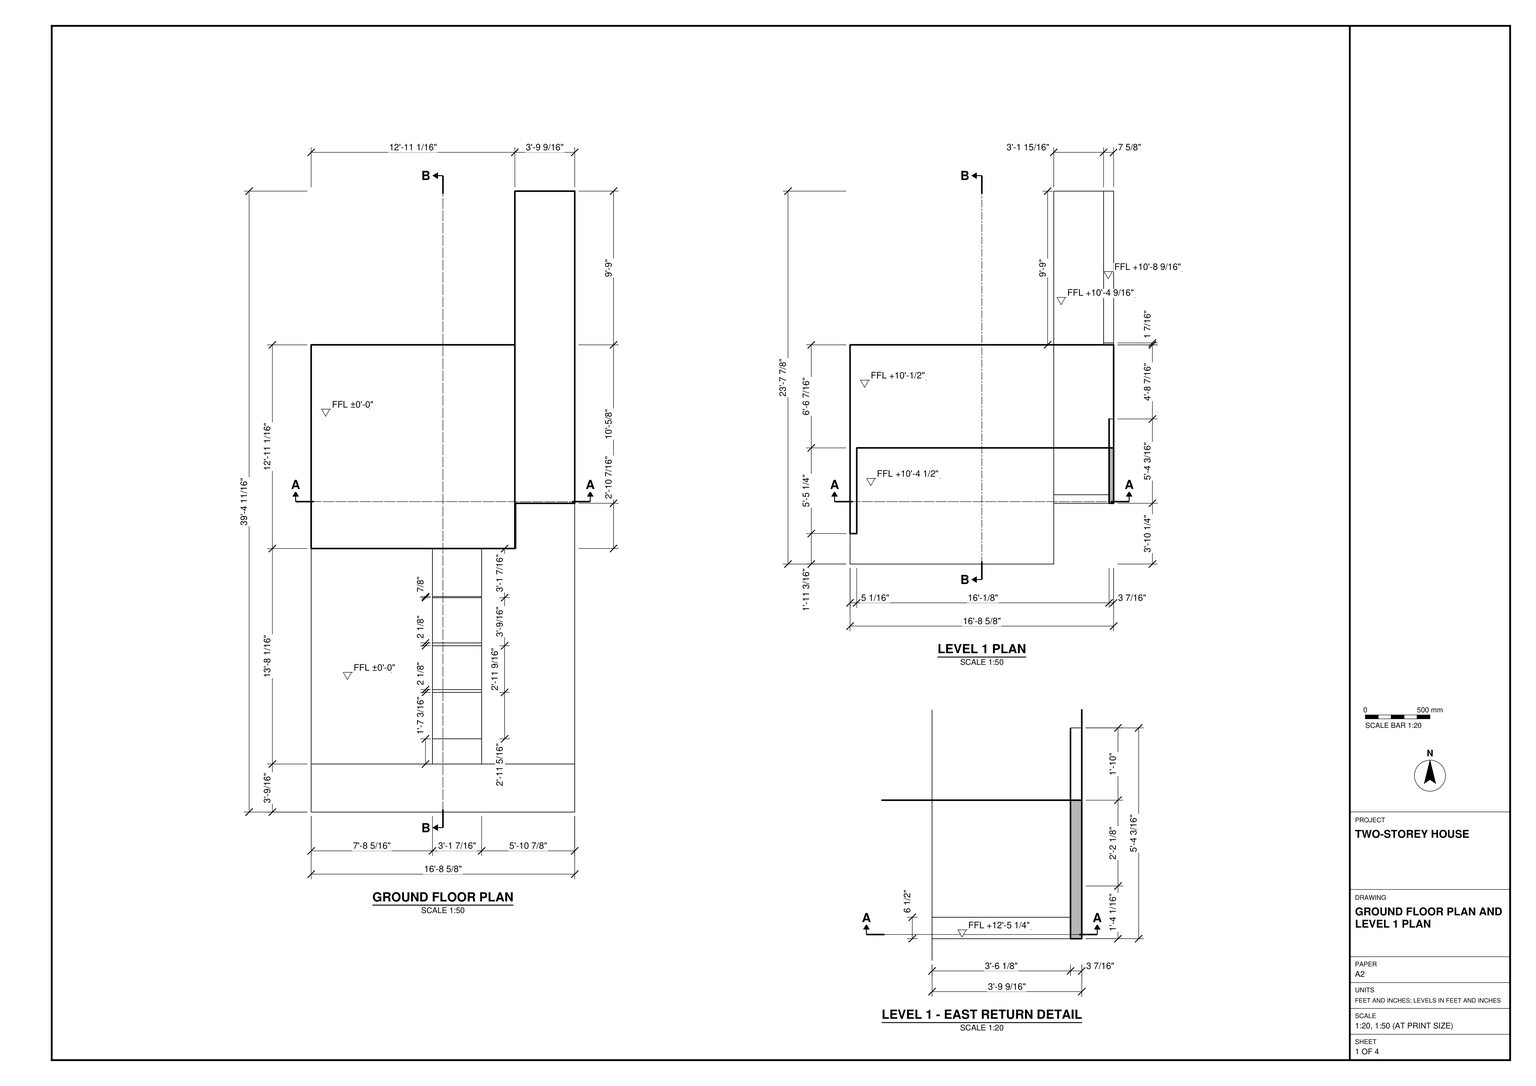
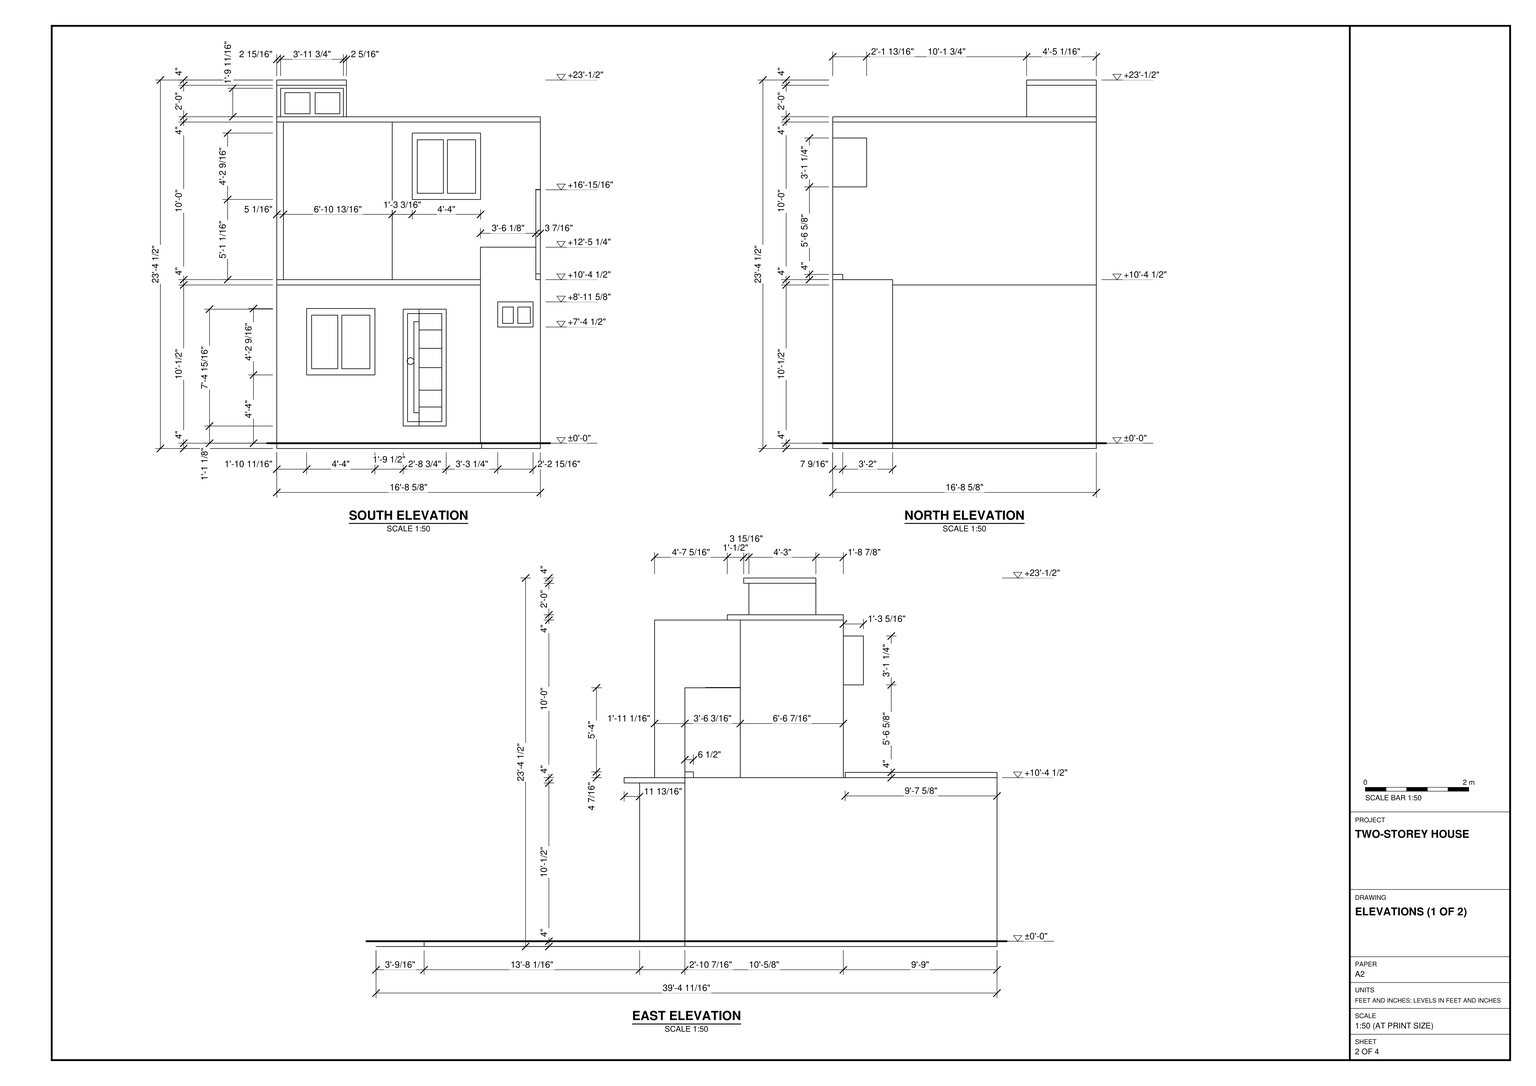
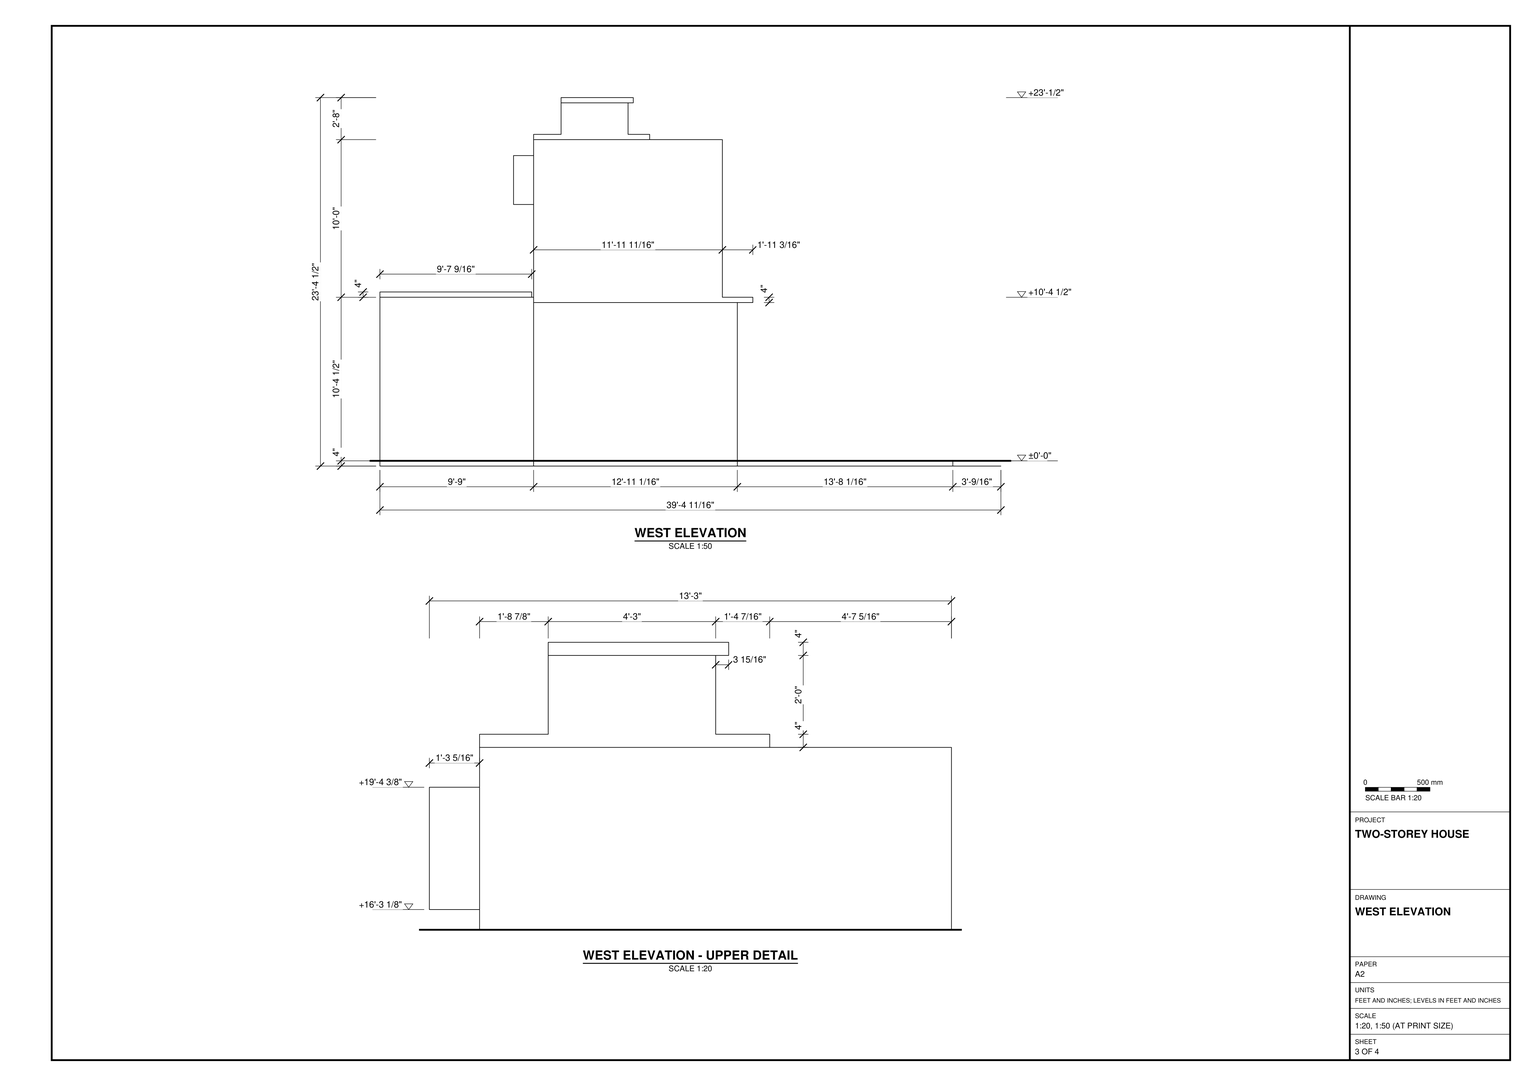
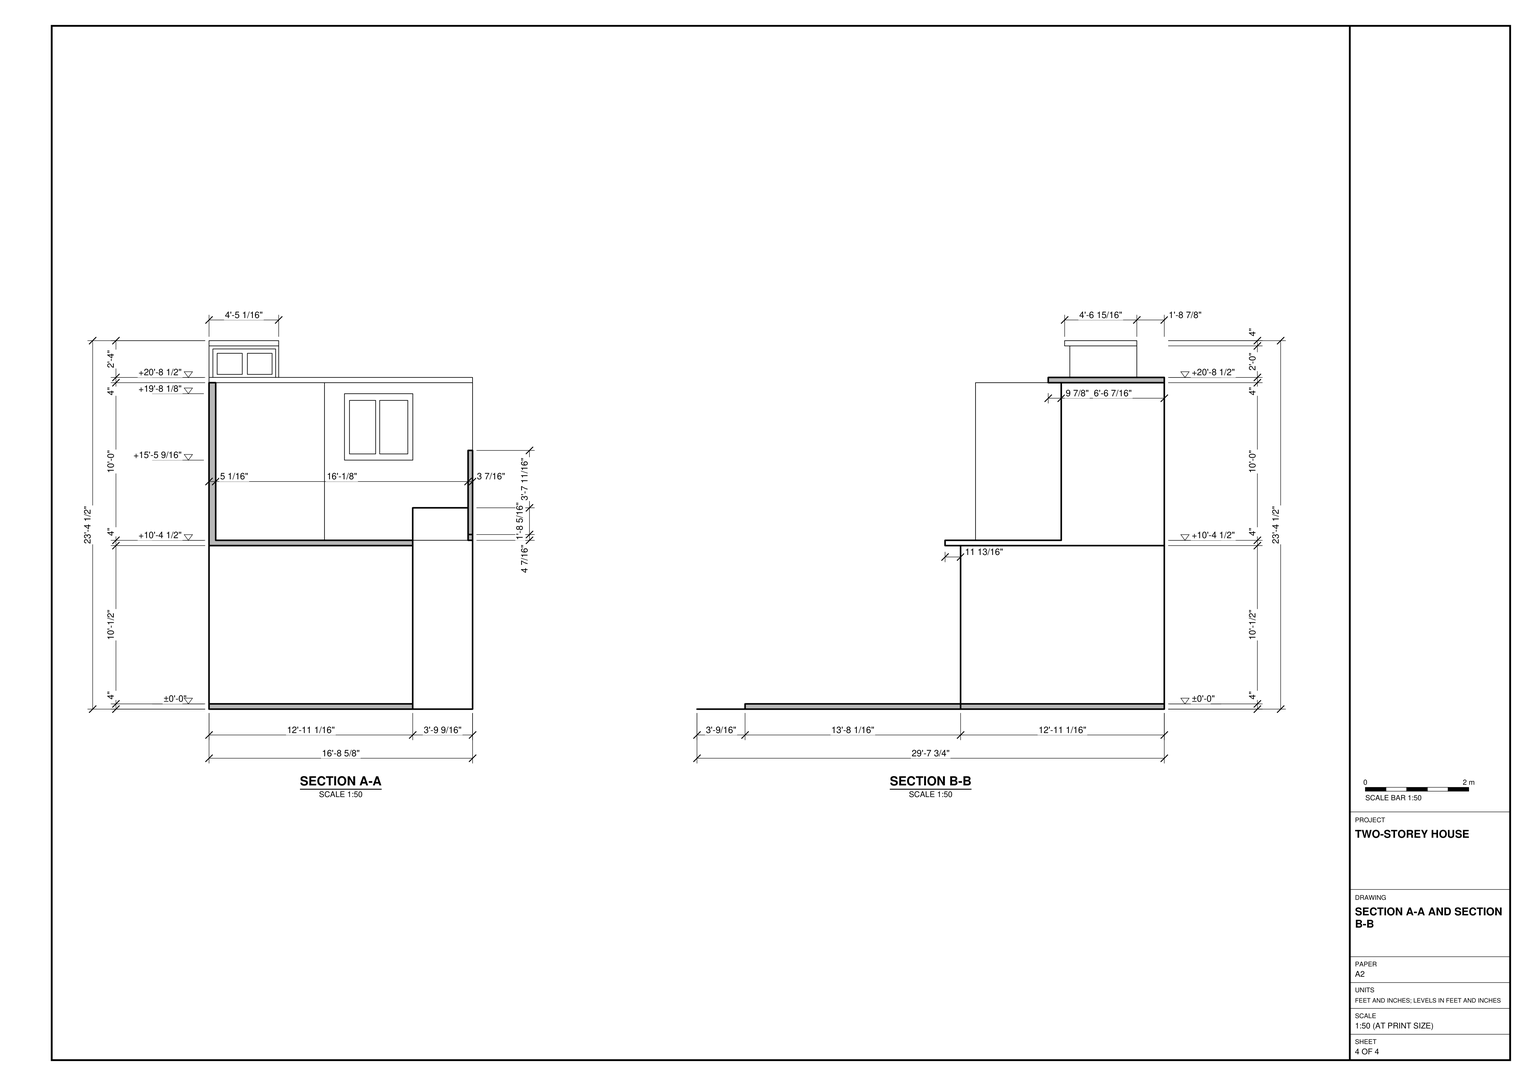
Build the two-storey house in SketchUp from task_files/diagram_01.pdf. Work in feet and inches. The overall model measures 16'-8 5/8" east to west, 39'-4 11/16" north to south and 23'-4 1/2" from the underside of the base to the top of the roof cap. Set the ground floor at ±0'-0" and Level 1 at +10'-4 1/2".

Use the ground-floor plan to lay out the base slab, the open approach on the south side, the main block and the narrow east wing that extends north beyond it. Include the divided strip in the approach. Follow the Level 1 plan for the upper walls, exposed slab edges and east return, using the wall thicknesses shown. On the south elevation, distinguish the entrance door, the paired window to its left and the smaller window on the east wing. Position the upper window independently of the lower openings. Match the flat roof profile, raised rooftop section and projecting cap to the elevations and enlarged detail.

Make walls, slabs and roof elements separate groups or components. Keep each furniture or joinery piece shown separate, and use components for repeated parts. Any decor or loose items may be suitable library components. Save one SketchUp model as output_files/two_storey_house_with_a_stepped_footprint_and_roof.skp.

# SketchUp Ruby script. Lengths in inches.
U = 1.inch
M = Sketchup.active_model
def pt(a) = Geom::Point3d.new(a.map { |v| v * U })
def face(e, loops, mat)
  f = e.add_face(loops[0].map { |a| pt(a) })
  loops[1..].each { |l| e.add_face(l.map { |a| pt(a) }).erase! }
  f.material = f.back_material = mat if mat
  f
end
# faces: each face lists its corners as indices into pts; further lists are holes
def faces(e, pts, list, mat = nil) = list.each { |f| face(e, (f[0].is_a?(Array) ? f : [f]).map { |l| l.map { |i| pts[i] } }, mat) }
# xy, xz, yz: faces in a plane at the given z, y or x. An outline is a flat list of corners, or four numbers for a rectangle; further outlines are holes
def ring(l) = l.size == 4 ? [[l[0], l[1]], [l[2], l[1]], [l[2], l[3]], [l[0], l[3]]] : l.each_slice(2).to_a
def flat(e, list, mat, &to3) = list.each { |f| face(e, (f[0].is_a?(Array) ? f : [f]).map { |l| ring(l).map { |u, v| to3.(u, v) } }, mat) }
def xy(e, z, list, mat = nil) = flat(e, list, mat) { |x, y| [x, y, z] }
def xz(e, y, list, mat = nil) = flat(e, list, mat) { |x, z| [x, y, z] }
def yz(e, x, list, mat = nil) = flat(e, list, mat) { |y, z| [x, y, z] }
def lines(e, pts, list) = list.each { |a, b| e.add_line(pt(pts[a]), pt(pts[b])) }
# prism: a flat outline (further loops are holes) pulled along v
def prism(e, loops, v, mat = nil)
  f = face(e, loops, mat); d = Geom::Vector3d.new(v.map { |x| x * U })
  f.pushpull(f.normal.samedirection?(d) ? d.length : -d.length)
end
def box(e, o, s, mat = nil) = prism(e, [[o, [o[0] + s[0], o[1], o[2]], [o[0] + s[0], o[1] + s[1], o[2]], [o[0], o[1] + s[1], o[2]]]], [0, 0, s[2]], mat)
def at(x, y, z, deg = 0) = Geom::Transformation.translation(pt([x, y, z])) * Geom::Transformation.rotation(ORIGIN, Z_AXIS, deg.degrees)
def axes(o, x, y, z) = Geom::Transformation.new([*x, 0, *y, 0, *z, 0, *pt(o).to_a, 1])
def part(name) = M.definitions.add(name)
# library, detail: a bought-in or finely detailed component or shape, given as its bounding box
def library(name, o, s) = part(name).tap { |d| box(d.entities, o, s) }
def detail(e, o, s) = box(e.add_group.entities, o, s)
def put(e, d, t, mat = nil) = e.add_instance(d, t).tap { |i| i.material = mat if mat }
def group(e, t, mat = nil) = e.add_group.tap { |g| g.transformation = t; g.material = mat if mat }.entities
root = M.entities
M.materials.add("C03_Honey_Glow").color = [255, 178, 101]
M.materials.add("C08_Toffee_Ember").color = [102, 51, 0]
M.materials.add("E01_Mint_Frost").color = [255, 255, 204]
M.materials.add("E08_Lime_Depth").color = [102, 102, 0]
M.materials.add("F08_Forest_Shadow").color = [51, 102, 0]
M.materials.add("Glass_Safety_01").color = [204, 235, 244]
M.materials["Glass_Safety_01"].alpha = 0.25
M.materials.add("Glass_Sky Reflection_01").color = [126, 138, 183]
M.materials["Glass_Sky Reflection_01"].alpha = 0.25
M.materials.add("M03_Pewter_Shine").color = [168, 168, 168]
M.materials.add("M04_Stone_Frost").color = [142, 142, 142]
M.materials.add("M05_Graphite_Haze").color = [114, 114, 114]
M.materials.add("M07_Charcoal_Gleam").color = [58, 58, 58]
M.materials.add("M09_Shadow_Night").color = [0, 0, 0]
M.materials.add("Metal_Perforated_03_1K").color = [205, 205, 205]
M.materials.add("Plywood_01_1K").color = [125, 96, 64]
xy(root,-4,[[0,36.59,155.98,200.66],[155.98,36.59,200.65,235.09]])
xy(root,-4,[[0,0,200.65,36.59]],"M09_Shadow_Night")
xy(root,0,[[0,36.59,92.33,200.66],[129.79,36.59,200.65,36.59,200.65,235.09,155.98,235.09,155.98,200.66,129.79,200.66]],"F08_Forest_Shadow")
xy(root,0,[[92.33,36.59,129.79,55.78],[92.33,55.78,129.79,91.09],[92.33,91.09,129.79,93.24],[92.33,93.24,129.79,126.63],[92.33,126.63,129.79,128.78],
  [92.33,128.78,129.79,163.2],[92.33,163.2,129.79,164.08],[92.33,164.08,129.79,200.66]],"Plywood_01_1K")
xy(root,128.54,[[193,357.16,200.65,472.71]])
xy(root,195.14,[[174.8125,355.72,200.65,371]])
xy(root,232.38,[[174.8125,355.72,200.65,371]])
xy(root,272.52,[[0,279.86,53.05,334.82]])
xy(root,276.52,[[0,279.86,53.05,334.82]],"M05_Graphite_Haze")
xz(root,36.59,[[0,-4,155.98,0],[155.98,-4,200.65,0]])
xz(root,200.66,[[0,-4,155.98,0]])
xz(root,235.09,[[155.98,-4,200.65,0]])
xz(root,279.86,[[0,272.52,53.05,276.52]])
xz(root,334.82,[[0,272.52,53.05,276.52]])
xz(root,355.72,[[174.8125,195.14,200.65,232.38]])
xz(root,357.16,[[193,124.54,200.65,128.54]])
xz(root,371,[[174.8125,195.14,200.65,232.38]])
xz(root,472.71,[[193,124.54,200.65,128.54]])
yz(root,0,[[36.59,-4,200.66,0],[279.86,272.52,334.82,276.52]])
yz(root,53.05,[[279.86,272.52,334.82,276.52]])
yz(root,155.98,[[200.66,-4,235.09,0]])
yz(root,174.8125,[[355.72,195.14,371,232.38]])
yz(root,193,[[355.72,124.52,472.71,124.52,472.71,124.54],[357.16,124.54,472.71,128.54]])
yz(root,200.65,[[36.59,-4,235.09,0],[357.16,124.54,472.71,128.54]])
yz(root,200.65,[[355.72,195.14,371,232.38]],"M03_Pewter_Shine")
p = [[200.65,355.72,124.52],[200.65,472.71,124.54],[193,472.71,124.54],[193,355.72,124.52],[197.28,251.125,130.34],[200.65,251.125,130.34],
  [193,355.72,124.54],[155.06,355.72,124.54],[155.06,472.71,124.54]]
faces(root,p,[[0,1,2,3]])
lines(root,p,[[4,5],[3,6],[6,7],[7,8],[8,2]])
g1 = group(root,at(0,200.66,-4))
box(g1,[0,0,0],[155.06,155.06,4])
g2 = group(root,at(0,200.66,0))
xy(g2,0,[[0,0,155.06,155.06]])
xy(g2,120.49,[[0,0,155.06,155.06]])
xz(g2,0,[[[0,0,155.06,120.49],[96.24,13.1,128.98,102.05],[22.71,52,74.74,102.58]],[99.57,16.43,108.34,16.43,108.34,23.19,104.4,23.19,104.4,62.52,104.3125,61.85,104.06,61.23,103.64,60.69,103.11,60.28,102.48,60.02,101.8125,59.93,101.14,60.02,100.52,60.28,99.98,60.69,99.57,61.23,99.57,61.24],[104.4,62.52,104.4,92.52,108.34,92.52,108.34,98.72,99.57,98.72,99.57,63.8,99.57,63.82,99.98,64.35,100.52,64.76,101.14,65.02,101.8125,65.11,102.48,65.02,103.11,64.76,103.64,64.35,104.06,63.82,104.3125,63.19]])
xz(g2,0,[[101.8125,59.93,102.48,60.02,103.11,60.28,103.64,60.69,104.06,61.23,104.3125,61.85,104.4,62.52,104.3125,63.19,104.06,63.82,103.64,64.35,103.11,64.76,102.48,65.02,101.8125,65.11,101.14,65.02,100.52,64.76,99.98,64.35,99.57,63.82,99.57,61.23,99.98,60.69,100.52,60.28,101.14,60.02]],"C08_Toffee_Ember")
xz(g2,0,[[108.34,16.43,125.65,27.57],[108.34,27.57,125.65,40.39],[108.34,40.39,125.65,57.58],[108.34,57.58,125.65,72.21],[108.34,72.21,125.65,86.26],
  [108.34,86.26,125.65,98.72]],"E01_Mint_Frost")
xz(g2,0,[[104.4,23.19,108.34,92.52]],"E08_Lime_Depth")
xz(g2,0,[[26.53,56.73,46.44,97.48],[49.51,56.73,70.91,97.48]],"Glass_Sky Reflection_01")
xz(g2,0,[[96.24,13.1,108.34,13.1,108.34,16.43,99.57,16.43,99.57,61.24,99.3125,61.85,99.23,62.52,99.3125,63.19,99.57,63.8,99.57,98.72,108.34,98.72,108.34,102.05,96.24,102.05],[108.34,13.1,128.98,13.1,128.98,102.05,108.34,102.05,108.34,98.72,125.65,98.72,125.65,16.43,108.34,16.43],[[22.71,52,74.74,102.58],[49.51,56.73,70.91,97.48],[26.53,56.73,46.44,97.48]],[99.57,61.24,99.57,63.8,99.3125,63.19,99.23,62.52,99.3125,61.85]],"M09_Shadow_Night")
xz(g2,155.06,[[0,0,155.06,120.49]])
yz(g2,0,[[0,0,155.06,120.49]])
yz(g2,155.06,[[0,0,155.06,120.49]])
g3 = group(root,at(155.06,206.6,-4),"Glass_Safety_01")
xy(g3,0,[[0,28.49,45.59,266.11]],"M04_Stone_Frost")
xy(g3,128.54,[[0,35.01,45.59,266.11]],"M04_Stone_Frost")
xy(g3,132.93,[[42.15,28.49,45.59,35.01]],"M04_Stone_Frost")
xy(g3,153.26,[[0,28.49,42.15,35.01]],"M04_Stone_Frost")
xz(g3,28.49,[[16.8125,95.25,25.01,107.69],[28.43,95.25,37.96,107.69]],"Glass_Safety_01")
xz(g3,28.49,[[[0,0,45.59,0,45.59,132.93,42.15,132.93,42.15,153.26,0,153.26],[13.14,92.49,40.06,111.62]]],"M04_Stone_Frost")
xz(g3,28.49,[[[13.14,92.49,40.06,111.62],[28.43,95.25,37.96,107.69],[16.8125,95.25,25.01,107.69]]],"M07_Charcoal_Gleam")
xz(g3,35.01,[[0,128.54,42.15,153.26],[42.15,128.54,45.59,132.93]],"M04_Stone_Frost")
xz(g3,266.11,[[0,0,45.59,128.54]],"M04_Stone_Frost")
yz(g3,0,[[28.49,0,28.49,153.26,35.01,153.26,35.01,128.54,266.11,128.54,266.11,0]],"M04_Stone_Frost")
yz(g3,42.15,[[28.49,132.93,35.01,153.26]],"M04_Stone_Frost")
yz(g3,45.59,[[28.49,0,266.11,0,266.11,128.54,35.01,128.54,35.01,132.93,28.49,132.93]],"M04_Stone_Frost")
g4 = group(root,at(0,188.83,120.49))
xy(g4,0,[[0,0,155.06,166.89]])
xy(g4,4.03,[[197.21,46.26,200.65,88.4375],[155.06,88.4375,155.06,166.89,200.65,166.89,200.65,110.45,197.21,110.45,197.21,88.4375],[197.21,88.4375,200.65,110.45]])
xy(g4,4.03,[[0,0,155.06,0,155.06,88.4375,5.08,88.4375,5.08,23.2,0,23.2]],"M05_Graphite_Haze")
xy(g4,72.45,[[197.21,46.26,200.65,62.29],[197.0625,62.29,197.21,88.4375],[197.21,62.29,200.65,88.4375]])
xy(g4,72.6875,[[197.0625,62.29,200.65,88.4375]])
xy(g4,124.03,[[0,23.2,5.08,88.4375],[0,88.4375,200.65,166.89]])
xz(g4,0,[[0,0,155.06,4.03]])
xz(g4,23.2,[[0,4.03,5.08,124.03]])
xz(g4,46.26,[[197.21,4.03,200.65,72.45]])
xz(g4,62.29,[[197.0625,72.45,200.65,72.6875]])
xz(g4,88.4375,[[[87.9,4.03,200.65,4.03,200.65,72.45,197.0625,72.45,197.0625,72.6875,200.65,72.6875,200.65,124.03,87.9,124.03],[103.12,65.07,155.15,115.65]]])
xz(g4,88.4375,[[5.08,4.03,87.9,124.03]],"C03_Honey_Glow")
xz(g4,88.4375,[[106.9375,69.8,126.85,110.55],[129.92,69.8,151.32,110.55]],"Glass_Safety_01")
xz(g4,88.4375,[[[103.12,65.07,155.15,115.65],[129.92,69.8,151.32,110.55],[106.9375,69.8,126.85,110.55]]],"M09_Shadow_Night")
xz(g4,166.89,[[0,0,0,124.03,200.65,124.03,200.65,4.03,155.06,4.03,155.06,0]])
yz(g4,0,[[0,0,0,4.03,23.2,4.03,23.2,124.03,166.89,124.03,166.89,0]])
yz(g4,5.08,[[23.2,4.03,88.4375,124.03]],"M05_Graphite_Haze")
yz(g4,155.06,[[0,0,166.89,4.03]])
yz(g4,197.0625,[[62.29,72.45,88.4375,72.6875]])
yz(g4,197.21,[[46.26,4.03,110.45,72.45]])
yz(g4,200.65,[[46.26,4.03,88.4375,72.45],[88.4375,4.03,166.89,4.03,166.89,124.03,88.4375,124.03,88.4375,72.6875,62.29,72.6875,62.29,72.45,88.4375,72.45]],"M03_Pewter_Shine")
p = [[197.21,110.45,72.45],[200.65,110.45,72.45]]
lines(g4,p,[[0,1]])
g5 = group(root,at(0,267.36,244.52),"M03_Pewter_Shine")
xy(g5,0,[[0,0,200.61,88.36]])
xy(g5,4,[[0,0,200.61,0,200.61,88.36,0,88.36,0,67.46,53.05,67.46,53.05,16.46,0,16.46]])
xy(g5,28,[[0,16.46,53.05,67.46]])
xz(g5,0,[[0,0,200.61,4]])
xz(g5,16.46,[[0,4,2.94,4,2.94,25.71,50.72,25.71,50.72,4,53.05,4,53.05,28,0,28]])
xz(g5,16.46,[[[2.94,4,50.72,25.71],[6.19,6.31,25.32,22.37],[29.21,6.31,48.01,22.37]]],"M09_Shadow_Night")
xz(g5,16.46,[[6.19,6.31,25.32,22.37],[29.21,6.31,48.01,22.37]],"Metal_Perforated_03_1K")
xz(g5,67.46,[[0,4,53.05,28]])
xz(g5,88.36,[[0,0,200.61,4]])
yz(g5,0,[[0,0,0,4,16.46,4,16.46,28,67.46,28,67.46,4,88.36,4,88.36,0]])
yz(g5,53.05,[[16.46,4,67.46,28]])
yz(g5,200.61,[[0,0,88.36,4]])
